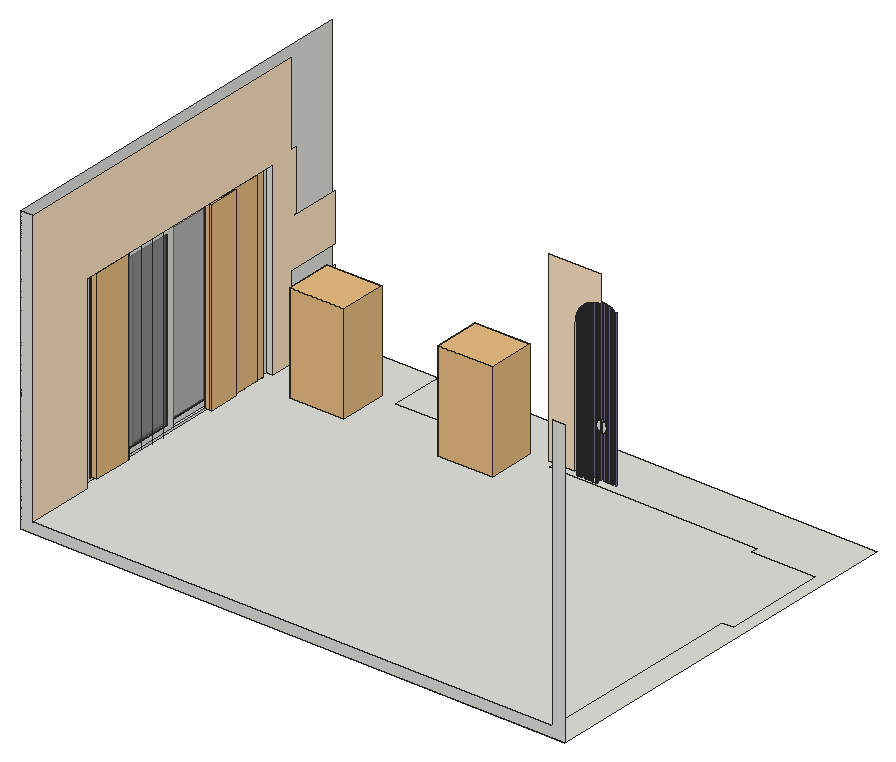
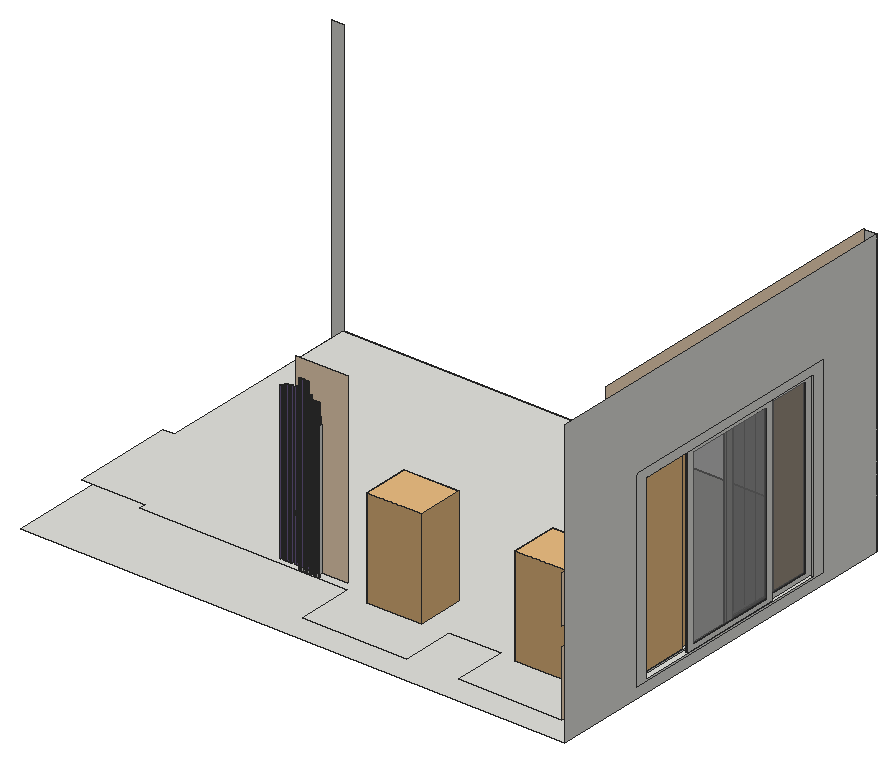
# SketchUp Ruby script. Lengths in inches.
U = 1.inch
M = Sketchup.active_model
def pt(a) = Geom::Point3d.new(a.map { |v| v * U })
def face(e, loops, mat)
  f = e.add_face(loops[0].map { |a| pt(a) })
  loops[1..].each { |l| e.add_face(l.map { |a| pt(a) }).erase! }
  f.material = f.back_material = mat if mat
  f
end
# faces: each face lists its corners as indices into pts; further lists are holes
def faces(e, pts, list, mat = nil) = list.each { |f| face(e, (f[0].is_a?(Array) ? f : [f]).map { |l| l.map { |i| pts[i] } }, mat) }
# xy, xz, yz: faces in a plane at the given z, y or x. An outline is a flat list of corners, or four numbers for a rectangle; further outlines are holes
def ring(l) = l.size == 4 ? [[l[0], l[1]], [l[2], l[1]], [l[2], l[3]], [l[0], l[3]]] : l.each_slice(2).to_a
def flat(e, list, mat, &to3) = list.each { |f| face(e, (f[0].is_a?(Array) ? f : [f]).map { |l| ring(l).map { |u, v| to3.(u, v) } }, mat) }
def xy(e, z, list, mat = nil) = flat(e, list, mat) { |x, y| [x, y, z] }
def xz(e, y, list, mat = nil) = flat(e, list, mat) { |x, z| [x, y, z] }
def yz(e, x, list, mat = nil) = flat(e, list, mat) { |y, z| [x, y, z] }
def lines(e, pts, list) = list.each { |a, b| e.add_line(pt(pts[a]), pt(pts[b])) }
# prism: a flat outline (further loops are holes) pulled along v
def prism(e, loops, v, mat = nil)
  f = face(e, loops, mat); d = Geom::Vector3d.new(v.map { |x| x * U })
  f.pushpull(f.normal.samedirection?(d) ? d.length : -d.length)
end
def box(e, o, s, mat = nil) = prism(e, [[o, [o[0] + s[0], o[1], o[2]], [o[0] + s[0], o[1] + s[1], o[2]], [o[0], o[1] + s[1], o[2]]]], [0, 0, s[2]], mat)
def at(x, y, z, deg = 0) = Geom::Transformation.translation(pt([x, y, z])) * Geom::Transformation.rotation(ORIGIN, Z_AXIS, deg.degrees)
def axes(o, x, y, z) = Geom::Transformation.new([*x, 0, *y, 0, *z, 0, *pt(o).to_a, 1])
def part(name) = M.definitions.add(name)
# library, detail: a bought-in or finely detailed component or shape, given as its bounding box
def library(name, o, s) = part(name).tap { |d| box(d.entities, o, s) }
def detail(e, o, s) = box(e.add_group.entities, o, s)
def put(e, d, t, mat = nil) = e.add_instance(d, t).tap { |i| i.material = mat if mat }
def group(e, t, mat = nil) = e.add_group.tap { |g| g.transformation = t; g.material = mat if mat }.entities
root = M.entities
M.materials.add("Carpet_Loop_Low").color = [201, 172, 127]
M.materials["Carpet_Loop_Low"].alpha = 0.3
M.materials.add("Translucent_Glass_Gray2").color = [128, 128, 128]
M.materials["Translucent_Glass_Gray2"].alpha = 0.5
M.materials.add("[0012_Bisque]").color = [255, 228, 196]
M.materials.add("[Color I01]").color = [116, 98, 147]
c1 = part("Curtain panel")
p = [[5.51,1.25,0],[5.9,0.93,0],[4.95,2.09,0],[5.1875,1.64,0],[6.35,0.69,0],[6.83,0.55,0],
  [7.33,0.5,0],[7.84,0.55,0],[8.32,0.69,0],[8.77,0.93,0],[9.16,1.25,0],[9.48,1.64,0],
  [9.72,2.09,0],[10,2.61,0],[10.375,3.0625,0],[10.83,3.4375,0],[17.64,0.16,0],[18.27,0.1,0],
  [11.35,3.71,0],[11.92,3.89,0],[12.51,3.94,0],[13.09,3.89,0],[20.56,1.04,0],[20.96,1.53,0],
  [13.66,3.71,0],[14.18,3.4375,0],[14.64,3.0625,0],[15.01,2.61,0],[15.29,2.09,0],[15.59,1.53,0],
  [15.99,1.04,0],[16.48,0.64,0],[17.04,0.34,0],[18.9,0.16,0],[19.51,0.34,0],[20.07,0.64,0],
  [21.26,2.09,0],[21.56,2.64,0],[21.96,3.13,0],[22.45,3.53,0],[23,3.83,0],[23.61,4.01,0],
  [24.24,4.08,0],[24.25,3.98,0]]
lines(c1.entities,p,[[0,1],[2,3],[3,0],[1,4],[4,5],[5,6],[6,7],[7,8],[8,9],[9,10],[10,11],[11,12],
  [12,13],[13,14],[14,15],[16,17],[15,18],[18,19],[19,20],[20,21],[22,23],[21,24],[24,25],[25,26],
  [26,27],[27,28],[28,29],[29,30],[30,31],[31,32],[32,16],[17,33],[33,34],[34,35],[35,22],[23,36],
  [36,37],[37,38],[38,39],[39,40],[40,41],[41,42],[42,43]])
detail(c1.entities,[0.85,0,0],[23.4,3.98,78.74])
c2 = part("Window frame")
prism(c2.entities,[[[7.875,28.35,0],[7.875,70.87,0],[7.875,70.87,47.24],[7.875,28.35,47.24]],[[7.875,68.9,0.38],[7.875,30.31,0.38],[7.875,30.31,45.28],[7.875,68.9,45.28]]],[-7.875,0,0])
c3 = part("Window sash")
xy(c3.entities,0,[[0,0,3.9375,16.73]])
xy(c3.entities,0.98,[[0,0.98,1.77,15.75],[1.77,0.98,2.85,15.75],[2.85,0.98,3.9375,15.75]])
xy(c3.entities,42.32,[[0,0.98,1.77,15.75],[1.77,0.98,2.85,15.75],[2.85,0.98,3.9375,15.75]])
xy(c3.entities,43.31,[[0,0,3.9375,16.73]])
xz(c3.entities,0,[[0,0,3.9375,43.31]])
xz(c3.entities,0.98,[[0,0.98,1.77,42.32],[1.77,0.98,2.85,42.32],[2.85,0.98,3.9375,42.32]])
xz(c3.entities,15.75,[[0,0.98,1.77,42.32],[1.77,0.98,2.85,42.32],[2.85,0.98,3.9375,42.32]])
xz(c3.entities,16.73,[[0,0,3.9375,43.31]])
yz(c3.entities,0,[[[0,0,16.73,43.31],[0.98,0.98,15.75,42.32]]])
yz(c3.entities,1.77,[[0.98,0.98,15.75,42.32]],"Translucent_Glass_Gray2")
yz(c3.entities,2.85,[[0.98,0.98,15.75,42.32]],"Translucent_Glass_Gray2")
yz(c3.entities,3.9375,[[[0,0,16.73,43.31],[0.98,0.98,15.75,42.32]]])
c4 = part("FoldingSlidingDoor3w")
g1 = group(c4.entities,at(-101.15,-5.12,-1))
put(g1,c2,axes([-4.6875,0,0],[0,-1.143,0],[2.15049,0,0],[0,0,1.73628]))
put(g1,c3,axes([101.99,-1.31,0.67],[0,-0.81153,0],[2.47938,0,0],[0,0,1.79978]))
put(g1,c3,axes([81.82,-4.5,0.67],[0,-0.81153,0],[2.47938,0,0],[0,0,1.79978]))
c5 = library("Component(2)\#6",[-17.32,-18.07,0.15],[16.9,14.46,30.65])
c6 = part("Group\#9")
xz(c6.entities,0,[[0.27,0,0.25,0.59,0.18,0.57,0.11,0.53,0.06,0.47,0.02,0.4,0,0.33,0,0.25,0.02,0.18,0.07,0.11,0.125,0.06,0.19,0.02],[0.35,0,0.42,0.02,0.49,0.07,0.54,0.125,0.58,0.19,0.6,0.27,0.59,0.35,0.57,0.42,0.53,0.49,0.47,0.54,0.4,0.58,0.33,0.6]])
xz(c6.entities,0.0625,[[0.27,0,0.35,0,0.33,0.6,0.25,0.59]])
yz(c6.entities,0,[[0,0.25,0.0625,0.33]])
p = [[0.125,0.0625,0.06],[0.19,0.0625,0.02],[0.19,0,0.02],[0.125,0,0.06],[0.27,0.0625,0],[0.27,0,0],
  [0.33,0.0625,0.6],[0.35,0.0625,0],[0.35,0,0],[0.33,0,0.6],[0.42,0.0625,0.02],[0.42,0,0.02],
  [0.25,0.0625,0.59],[0.25,0,0.59],[0.49,0.0625,0.07],[0.49,0,0.07],[0.02,0.0625,0.18],[0.07,0.0625,0.11],
  [0.07,0,0.11],[0.02,0,0.18],[0.54,0.0625,0.125],[0.54,0,0.125],[0.58,0.0625,0.19],[0.58,0,0.19],
  [0,0.0625,0.25],[0,0,0.25],[0.6,0.0625,0.27],[0.6,0,0.27],[0.02,0.0625,0.4],[0,0.0625,0.33],
  [0,0,0.33],[0.02,0,0.4],[0.59,0.0625,0.35],[0.57,0.0625,0.42],[0.57,0,0.42],[0.59,0,0.35],
  [0.06,0.0625,0.47],[0.06,0,0.47],[0.53,0.0625,0.49],[0.53,0,0.49],[0.18,0.0625,0.57],[0.11,0.0625,0.53],
  [0.11,0,0.53],[0.18,0,0.57],[0.47,0.0625,0.54],[0.4,0.0625,0.58],[0.4,0,0.58],[0.47,0,0.54]]
faces(c6.entities,p,[[0,1,2,3],[1,4,5,2],[6,7,8,9],[7,10,11,8],[4,12,13,5],[10,14,15,11],[16,17,18,19],[17,0,3,18],
  [14,20,21,15],[20,22,23,21],[24,16,19,25],[22,26,27,23],[28,29,30,31],[32,33,34,35],[26,32,35,27],[36,28,31,37],
  [33,38,39,34],[40,41,42,43],[41,36,37,42],[44,45,46,47],[38,44,47,39],[12,40,43,13],[45,6,9,46]])
xy(root,0,[[0,0,238.375,170.3125]])
xy(root,4.6875,[[5.62,0,233.26,0,233.26,92.18,238.375,92.18,238.375,136.82,210.45,136.82,210.45,139.88,119.1875,139.88,119.1875,164.88,73.56,164.88,73.56,141.7,50.74,141.7,50.74,164.88,5.62,164.88,5.62,131.05,0,131.05,0,29.49,5.62,29.49]])
xz(root,0,[[0,0,238.375,0,238.375,124.6875,233.26,124.6875,233.26,4.6875,5.62,4.6875,5.62,118.75,4.82,118.75,4.82,124.6875,0,124.6875]])
xz(root,29.49,[[0,4.6875,0,88.0625,2.71,88.0625,2.71,87,5.62,87,5.62,4.6875]])
xz(root,131.05,[[0,4.6875,5.62,4.6875,5.62,87,2.71,87,2.71,88.0625,0,88.0625]])
xz(root,139.88,[[119.1875,7.1875,130.59,7.1875,130.59,65.41,130.61,66.01,130.63,66.31,130.69,66.91,130.73,67.2,130.79,67.5,130.84,67.79,130.91,68.09,130.98,68.38,131.0625,68.67,131.15,68.95,131.25,69.24,131.35,69.52,131.46,69.8,131.58,70.07,131.7,70.35,131.83,70.62,131.97,70.88,132.12,71.15,132.27,71.4,132.43,71.66,132.59,71.91,132.77,72.16,132.94,72.4,133.13,72.63,133.32,72.87,133.52,73.09,133.72,73.3125,133.93,73.53,134.14,73.74,134.36,73.95,134.58,74.15,134.8125,74.34,135.05,74.53,135.29,74.71,135.53,74.88,136.03,75.22,136.55,75.52,136.8125,75.66,137.08,75.8,137.35,75.93,137.625,76.05,137.9,76.16,138.18,76.27,138.47,76.37,138.75,76.46,139.33,76.62,139.62,76.69,139.92,76.75,140.21,76.81,140.51,76.85,140.8,76.89,141.4,76.95,141.7,76.96,142,76.95,142,88.4375,119.1875,88.4375]],"[0012_Bisque]")
xz(root,140.54,[[131.36,5.5,131.4375,7.1875],[131.4375,5.5,131.52,7.1875],[133.05,5.5,133.125,7.1875],[133.125,5.5,133.2,7.1875],[134.74,5.5,134.8125,7.1875],
  [134.8125,5.5,134.89,7.1875],[136.42,5.5,136.5,7.1875],[136.5,5.5,136.58,7.1875],[138.05,5.5,138.125,7.1875],[138.125,5.5,138.2,7.1875],
  [139.67,5.5,139.75,7.1875],[139.75,5.5,139.83,7.1875]])
xz(root,140.54,[[131.36,7.1875,131.4375,74.15],[131.4375,7.1875,131.52,74.15],[133.05,7.1875,133.125,74.15],[133.125,7.1875,133.2,74.15],[134.74,7.1875,134.8125,75.9375],
  [134.8125,7.1875,134.89,75.9375],[136.42,7.1875,136.5,80.75],[136.5,7.1875,136.58,80.75],[138.05,7.1875,138.125,80.75],[138.125,7.1875,138.2,80.75],
  [139.67,7.1875,139.75,80.75],[139.75,7.1875,139.83,80.75]],"[Color I01]")
yz(root,0,[[[0,0,170.3125,124.6875],[29.49,4.6875,131.05,88.0625]]])
yz(root,5.62,[[0,4.6875,29.49,4.6875,29.49,87,131.05,87,131.05,4.6875,164.88,4.6875,164.88,33.18,141.2,33.18,141.2,41.1875,164.88,41.1875,164.88,62.0625,142.63,62.0625,142.63,62.625,143.84,62.625,143.84,88.4375,141.2,88.4375,141.2,124.6875,0,124.6875]],"[0012_Bisque]")
yz(root,130.59,[[139.88,7.1875,141.2,65.41]])
p = [[131.29,140.55,5.5],[131.36,140.54,5.5],[131.36,140.54,7.1875],[131.29,140.55,7.1875],[131.52,140.54,5.5],[131.59,140.55,5.5],
  [131.59,140.55,7.1875],[131.52,140.54,7.1875],[132.97,140.55,5.5],[133.05,140.54,5.5],[133.05,140.54,7.1875],[132.97,140.55,7.1875],
  [133.2,140.54,5.5],[133.28,140.55,5.5],[133.28,140.55,7.1875],[133.2,140.54,7.1875],[134.66,140.55,5.5],[134.74,140.54,5.5],
  [134.74,140.54,7.1875],[134.66,140.55,7.1875],[134.89,140.54,5.5],[134.97,140.55,5.5],[134.97,140.55,7.1875],[134.89,140.54,7.1875],
  [136.35,140.55,5.5],[136.42,140.54,5.5],[136.42,140.54,7.1875],[136.35,140.55,7.1875],[136.58,140.54,5.5],[136.65,140.55,5.5],
  [136.65,140.55,7.1875],[136.58,140.54,7.1875],[137.97,140.55,5.5],[138.05,140.54,5.5],[138.05,140.54,7.1875],[137.97,140.55,7.1875],
  [138.2,140.54,5.5],[138.28,140.55,5.5],[138.28,140.55,7.1875],[138.2,140.54,7.1875],[139.6,140.55,5.5],[139.67,140.54,5.5],
  [139.67,140.54,7.1875],[139.6,140.55,7.1875],[139.83,140.54,5.5],[139.9,140.55,5.5],[139.9,140.55,7.1875],[139.83,140.54,7.1875],
  [131,140.66,5.5],[131.07,140.625,5.5],[131.07,140.625,7.1875],[131,140.66,7.1875],[131.14,140.59,5.5],[131.21,140.57,5.5],
  [131.21,140.57,7.1875],[131.14,140.59,7.1875],[131.67,140.57,5.5],[131.67,140.57,7.1875],[131.74,140.59,5.5],[131.74,140.59,7.1875],
  [131.81,140.625,5.5],[131.81,140.625,7.1875],[131.88,140.66,5.5],[131.88,140.66,7.1875],[132.6875,140.66,5.5],[132.75,140.625,5.5],
  [132.75,140.625,7.1875],[132.6875,140.66,7.1875],[132.83,140.59,5.5],[132.9,140.57,5.5],[132.9,140.57,7.1875],[132.83,140.59,7.1875],
  [133.35,140.57,5.5],[133.35,140.57,7.1875],[133.43,140.59,5.5],[133.43,140.59,7.1875],[133.5,140.625,5.5],[133.5,140.625,7.1875],
  [133.57,140.66,5.5],[133.57,140.66,7.1875],[134.44,140.625,5.5],[134.51,140.59,5.5],[134.51,140.59,7.1875],[134.44,140.625,7.1875],
  [134.375,140.66,5.5],[134.375,140.66,7.1875],[134.59,140.57,5.5],[134.59,140.57,7.1875],[135.04,140.57,5.5],[135.04,140.57,7.1875],
  [135.11,140.59,5.5],[135.11,140.59,7.1875],[135.18,140.625,5.5],[135.18,140.625,7.1875],[135.25,140.66,5.5],[135.25,140.66,7.1875],
  [136.13,140.625,5.5],[136.2,140.59,5.5],[136.2,140.59,7.1875],[136.13,140.625,7.1875],[136.0625,140.66,5.5],[136.0625,140.66,7.1875],
  [136.27,140.57,5.5],[136.27,140.57,7.1875],[136.73,140.57,5.5],[136.73,140.57,7.1875],[136.8,140.59,5.5],[136.8,140.59,7.1875],
  [136.87,140.625,5.5],[136.87,140.625,7.1875],[136.94,140.66,5.5],[136.94,140.66,7.1875],[137.6875,140.66,5.5],[137.75,140.625,5.5],
  [137.75,140.625,7.1875],[137.6875,140.66,7.1875],[137.83,140.59,5.5],[137.9,140.57,5.5],[137.9,140.57,7.1875],[137.83,140.59,7.1875],
  [138.35,140.57,5.5],[138.35,140.57,7.1875],[138.43,140.59,5.5],[138.43,140.59,7.1875],[138.5,140.625,5.5],[138.5,140.625,7.1875],
  [138.57,140.66,5.5],[138.57,140.66,7.1875],[139.3125,140.66,5.5],[139.38,140.625,5.5],[139.38,140.625,7.1875],[139.3125,140.66,7.1875],
  [139.45,140.59,5.5],[139.45,140.59,7.1875],[139.52,140.57,5.5],[139.52,140.57,7.1875],[139.98,140.57,5.5],[139.98,140.57,7.1875],
  [140.05,140.59,5.5],[140.05,140.59,7.1875],[140.12,140.625,5.5],[140.12,140.625,7.1875],[140.19,140.66,5.5],[140.19,140.66,7.1875],
  [130.82,140.8,5.5],[130.875,140.75,5.5],[130.875,140.75,7.1875],[130.82,140.8,7.1875],[130.93,140.7,5.5],[130.93,140.7,7.1875],
  [131.94,140.7,5.5],[131.94,140.7,7.1875],[132,140.75,5.5],[132,140.75,7.1875],[132.06,140.8,5.5],[132.06,140.8,7.1875],
  [132.51,140.8,5.5],[132.5625,140.75,5.5],[132.5625,140.75,7.1875],[132.51,140.8,7.1875],[132.62,140.7,5.5],[132.62,140.7,7.1875],
  [133.63,140.7,5.5],[133.63,140.7,7.1875],[133.69,140.75,5.5],[133.69,140.75,7.1875],[134.25,140.75,5.5],[134.31,140.7,5.5],
  [134.31,140.7,7.1875],[134.25,140.75,7.1875],[135.32,140.7,5.5],[135.32,140.7,7.1875],[135.38,140.75,5.5],[135.38,140.75,7.1875],
  [135.9375,140.75,5.5],[136,140.7,5.5],[136,140.7,7.1875],[135.9375,140.75,7.1875],[137,140.7,5.5],[137,140.7,7.1875],
  [137.07,140.75,5.5],[137.07,140.75,7.1875],[137.62,140.7,5.5],[137.62,140.7,7.1875],[137.5625,140.75,5.5],[137.5625,140.75,7.1875],
  [138.63,140.7,5.5],[138.63,140.7,7.1875],[138.69,140.75,5.5],[138.69,140.75,7.1875],[139.25,140.7,5.5],[139.25,140.7,7.1875],
  [139.1875,140.75,5.5],[139.1875,140.75,7.1875],[140.25,140.7,5.5],[140.25,140.7,7.1875],[140.32,140.75,5.5],[140.32,140.75,7.1875],
  [131.29,140.55,74.15],[131.36,140.54,74.15],[131.52,140.54,74.15],[131.59,140.55,74.15],[132.97,140.55,74.15],[133.05,140.54,74.15],
  [133.2,140.54,74.15],[133.28,140.55,74.15],[134.66,140.55,75.9375],[134.74,140.54,75.9375],[134.89,140.54,75.9375],[134.97,140.55,75.9375],
  [136.35,140.55,80.75],[136.42,140.54,80.75],[136.58,140.54,80.75],[136.65,140.55,80.75],[137.97,140.55,80.75],[138.05,140.54,80.75],
  [138.2,140.54,80.75],[138.28,140.55,80.75],[139.6,140.55,80.75],[139.67,140.54,80.75],[139.83,140.54,80.75],[139.9,140.55,80.75],
  [131,140.66,74.15],[131.07,140.625,74.15],[131.14,140.59,74.15],[131.21,140.57,74.15],[131.67,140.57,74.15],[131.74,140.59,74.15],
  [131.81,140.625,74.15],[131.88,140.66,74.15],[132.6875,140.66,74.15],[132.75,140.625,74.15],[132.83,140.59,74.15],[132.9,140.57,74.15],
  [133.35,140.57,74.15],[133.43,140.59,74.15],[133.5,140.625,74.15],[133.57,140.66,74.15],[134.44,140.625,75.9375],[134.51,140.59,75.9375],
  [134.375,140.66,75.9375],[134.59,140.57,75.9375],[135.04,140.57,75.9375],[135.11,140.59,75.9375],[135.18,140.625,75.9375],[135.25,140.66,75.9375],
  [136.13,140.625,80.75],[136.2,140.59,80.75],[136.0625,140.66,80.75],[136.27,140.57,80.75],[136.73,140.57,80.75],[136.8,140.59,80.75],
  [136.87,140.625,80.75],[136.94,140.66,80.75],[137.6875,140.66,80.75],[137.75,140.625,80.75],[137.83,140.59,80.75],[137.9,140.57,80.75],
  [138.35,140.57,80.75],[138.43,140.59,80.75],[138.5,140.625,80.75],[138.57,140.66,80.75],[139.3125,140.66,80.75],[139.38,140.625,80.75],
  [139.45,140.59,80.75],[139.52,140.57,80.75],[139.98,140.57,80.75],[140.05,140.59,80.75],[140.12,140.625,80.75],[140.19,140.66,80.75],
  [140.85,140.71,76.87],[140.85,140.71,7.1875],[141,140.64,7.1875],[141,140.64,76.87],[141.16,140.6,7.1875],[141.16,140.6,76.87],
  [141.32,140.59,7.1875],[141.32,140.59,76.87],[141.48,140.62,7.1875],[141.48,140.62,76.87],[141.63,140.68,7.1875],[141.63,140.68,76.87],
  [130.82,140.8,74.15],[130.875,140.75,74.15],[130.93,140.7,74.15],[131.94,140.7,74.15],[132,140.75,74.15],[132.06,140.8,74.15],
  [132.62,140.7,74.15],[132.5625,140.75,74.15],[133.63,140.7,74.15],[133.69,140.75,74.15],[134.25,140.75,75.9375],[134.31,140.7,75.9375],
  [135.32,140.7,75.9375],[135.38,140.75,75.9375],[135.9375,140.75,80.75],[136,140.7,80.75],[137,140.7,80.75],[137.07,140.75,80.75],
  [137.62,140.7,80.75],[137.5625,140.75,80.75],[138.63,140.7,80.75],[138.69,140.75,80.75],[139.25,140.7,80.75],[139.1875,140.75,80.75],
  [140.25,140.7,80.75],[140.32,140.75,80.75],[140.73,140.82,76.87],[140.73,140.82,7.1875],[141.77,140.78,7.1875],[141.77,140.78,76.87],
  [142.57,140.74,76.91],[142.57,140.74,7.1875],[142.7,140.68,7.1875],[142.7,140.68,76.91],[142.83,140.67,7.1875],[142.83,140.67,76.91],
  [142.97,140.68,7.1875],[142.97,140.68,76.91],[143.1,140.74,7.1875],[143.1,140.74,76.91],[143.63,140.74,76.75],[143.63,140.74,7.1875],
  [143.76,140.68,7.1875],[143.76,140.68,76.75],[143.9,140.67,7.1875],[143.9,140.67,76.75],[144.03,140.68,7.1875],[144.03,140.68,76.75],
  [144.16,140.74,7.1875],[144.16,140.74,76.75],[144.69,140.74,76.48],[144.69,140.74,7.1875],[144.82,140.68,7.1875],[144.82,140.68,76.48],
  [144.96,140.67,7.1875],[144.96,140.67,76.48],[145.1,140.68,7.1875],[145.1,140.68,76.48],[145.22,140.74,7.1875],[145.22,140.74,76.48],
  [145.76,140.74,76.1],[145.76,140.74,7.1875],[145.88,140.68,7.1875],[145.88,140.68,76.1],[146.02,140.67,7.1875],[146.02,140.67,76.1],
  [146.16,140.68,7.1875],[146.16,140.68,76.1],[146.29,140.74,7.1875],[146.29,140.74,76.1],[146.82,140.74,75.6],[146.82,140.74,7.1875],
  [146.95,140.68,7.1875],[146.95,140.68,75.6],[147.08,140.67,7.1875],[147.08,140.67,75.6],[147.22,140.68,7.1875],[147.22,140.68,75.6],
  [147.35,140.74,7.1875],[147.35,140.74,75.6],[147.88,140.74,74.96],[147.88,140.74,7.1875],[148.01,140.68,7.1875],[148.01,140.68,74.96],
  [148.15,140.67,7.1875],[148.15,140.67,74.96],[148.28,140.68,7.1875],[148.28,140.68,74.96],[148.41,140.74,7.1875],[148.41,140.74,74.96],
  [4.7,104.82,86.88],[4.7,104.82,6.18],[4.51,104.95,6.18],[4.51,104.95,86.88],[5.32,110.01,6.18],[5.32,110.01,86.88],
  [5.51,115.55,86.88],[5.51,115.55,6.18],[5.62,96.58,6.18],[5.62,96.58,86.88],[4.51,60.63,6.18],[4.51,60.63,86.88],
  [5.62,52.27,6.18],[5.62,52.27,86.88],[4.7,60.5,86.88],[4.7,60.5,6.18],[5.51,71.23,86.88],[5.51,71.23,6.18],
  [5.32,65.69,6.18],[5.32,65.69,86.88]]
faces(root,p,[[0,1,2,3],[4,5,6,7],[8,9,10,11],[12,13,14,15],[16,17,18,19],[20,21,22,23],[24,25,26,27],[28,29,30,31],
  [32,33,34,35],[36,37,38,39],[40,41,42,43],[44,45,46,47],[48,49,50,51],[52,53,54,55],[49,52,55,50],[53,0,3,54],
  [5,56,57,6],[56,58,59,57],[58,60,61,59],[60,62,63,61],[64,65,66,67],[68,69,70,71],[65,68,71,66],[69,8,11,70],
  [13,72,73,14],[72,74,75,73],[74,76,77,75],[76,78,79,77],[80,81,82,83],[84,80,83,85],[81,86,87,82],[86,16,19,87],
  [21,88,89,22],[88,90,91,89],[90,92,93,91],[92,94,95,93],[96,97,98,99],[100,96,99,101],[97,102,103,98],[102,24,27,103],
  [29,104,105,30],[104,106,107,105],[106,108,109,107],[108,110,111,109],[112,113,114,115],[116,117,118,119],[113,116,119,114],[117,32,35,118],
  [37,120,121,38],[120,122,123,121],[122,124,125,123],[124,126,127,125],[128,129,130,131],[129,132,133,130],[134,40,43,135],[132,134,135,133],
  [45,136,137,46],[136,138,139,137],[138,140,141,139],[140,142,143,141],[144,145,146,147],[148,48,51,149],[145,148,149,146],[62,150,151,63],
  [150,152,153,151],[152,154,155,153],[156,157,158,159],[160,64,67,161],[157,160,161,158],[78,162,163,79],[162,164,165,163],[166,167,168,169],
  [167,84,85,168],[94,170,171,95],[170,172,173,171],[174,175,176,177],[175,100,101,176],[110,178,179,111],[178,180,181,179],[182,112,115,183],
  [184,182,183,185],[126,186,187,127],[186,188,189,187],[190,128,131,191],[192,190,191,193],[142,194,195,143],[194,196,197,195]])
faces(root,p,[[198,3,2,199],[200,7,6,201],[202,11,10,203],[204,15,14,205],[206,19,18,207],[208,23,22,209],[210,27,26,211],[212,31,30,213],
  [214,35,34,215],[216,39,38,217],[218,43,42,219],[220,47,46,221],[222,51,50,223],[224,55,54,225],[223,50,55,224],[225,54,3,198],
  [201,6,57,226],[226,57,59,227],[227,59,61,228],[228,61,63,229],[230,67,66,231],[232,71,70,233],[231,66,71,232],[233,70,11,202],
  [205,14,73,234],[234,73,75,235],[235,75,77,236],[236,77,79,237],[238,83,82,239],[240,85,83,238],[239,82,87,241],[241,87,19,206],
  [209,22,89,242],[242,89,91,243],[243,91,93,244],[244,93,95,245],[246,99,98,247],[248,101,99,246],[247,98,103,249],[249,103,27,210],
  [213,30,105,250],[250,105,107,251],[251,107,109,252],[252,109,111,253],[254,115,114,255],[256,119,118,257],[255,114,119,256],[257,118,35,214],
  [217,38,121,258],[258,121,123,259],[259,123,125,260],[260,125,127,261],[262,131,130,263],[263,130,133,264],[265,135,43,218],[264,133,135,265],
  [221,46,137,266],[266,137,139,267],[267,139,141,268],[268,141,143,269],[270,271,272,273],[273,272,274,275],[275,274,276,277],[277,276,278,279],
  [279,278,280,281],[282,147,146,283],[284,149,51,222],[283,146,149,284],[229,63,151,285],[285,151,153,286],[286,153,155,287],[288,161,67,230],
  [289,158,161,288],[237,79,163,290],[290,163,165,291],[292,169,168,293],[293,168,85,240],[245,95,171,294],[294,171,173,295],[296,177,176,297],
  [297,176,101,248],[253,111,179,298],[298,179,181,299],[300,183,115,254],[301,185,183,300],[261,127,187,302],[302,187,189,303],[304,191,131,262],
  [305,193,191,304],[269,143,195,306],[306,195,197,307],[308,309,271,270],[281,280,310,311],[312,313,314,315],[315,314,316,317],[317,316,318,319],
  [319,318,320,321],[322,323,324,325],[325,324,326,327],[327,326,328,329],[329,328,330,331],[332,333,334,335],[335,334,336,337],[337,336,338,339],
  [339,338,340,341],[342,343,344,345],[345,344,346,347],[347,346,348,349],[349,348,350,351],[352,353,354,355],[355,354,356,357],[357,356,358,359],
  [359,358,360,361],[362,363,364,365],[365,364,366,367],[367,366,368,369],[369,368,370,371]],"[Color I01]")
lines(root,p,[[372,373],[374,375],[376,377],[378,379],[380,381],[382,383],[384,385],[386,387],[388,389],[390,391]])
put(root,c1,axes([2.87,34.17,6.18],[0,0.74645,0],[0.6902,0,0],[0,0,1.02495]),"Carpet_Loop_Low")
put(root,c4,axes([4.25,81.2,5.7],[0,-1.11073,0],[0.30123,0,0],[0,0,1.01641]))
put(root,c1,axes([3.65,96.11,6.18],[0,0.56283,0],[0.6902,0,0],[0,0,1.02495]),"Carpet_Loop_Low")
put(root,c1,axes([2.83,101.96,6.18],[0,0.98919,0],[0.6902,0,0],[0,0,1.02495]),"Carpet_Loop_Low")
put(root,c1,axes([2.87,108.64,6.18],[0,0.56283,0],[0.6902,0,0],[0,0,1.02495]),"Carpet_Loop_Low")
put(root,c5,axes([19.28,117.43,4.47],[-1.41,0,0],[0,-1.41,0],[0,0,1.41]))
put(root,c5,axes([84.16,117.43,4.47],[-1.41,0,0],[0,-1.41,0],[0,0,1.41]))
put(root,c6,axes([139.77,140.2,26.13],[7.7976,0,0],[0,7.7976,0],[0,0,7.7976]))
